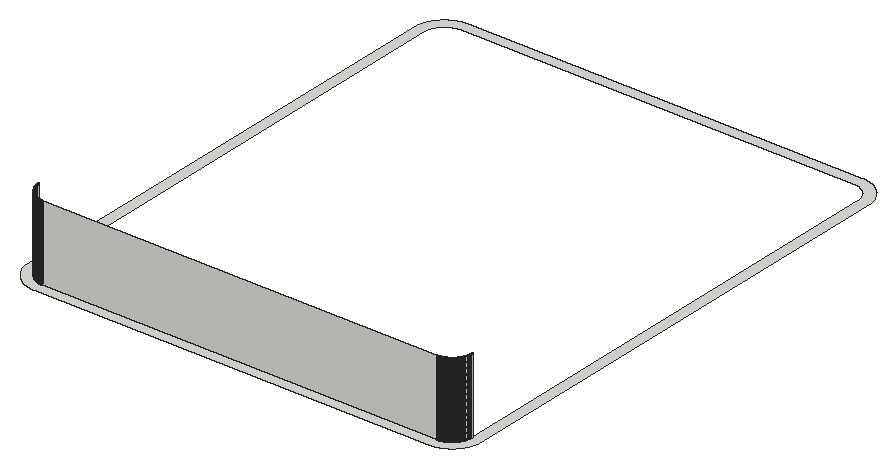
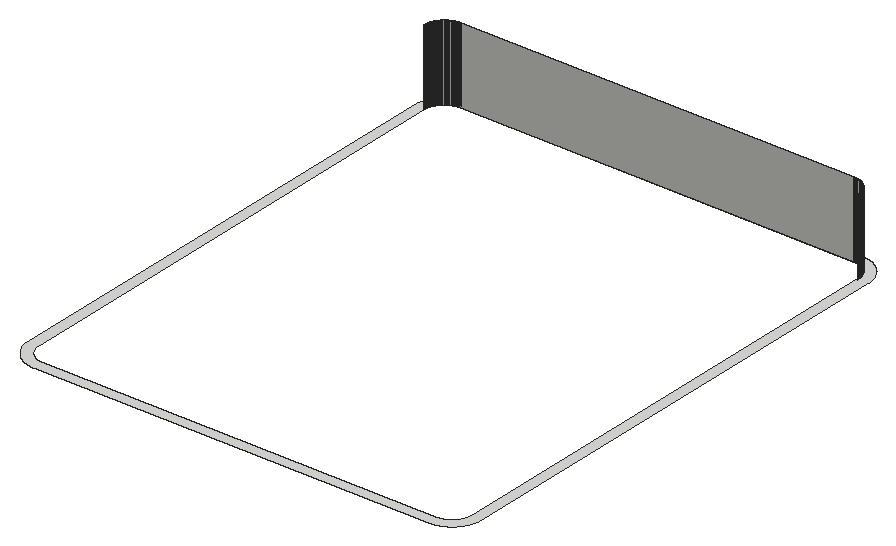
# SketchUp Ruby script. Lengths in inches.
U = 1.inch
M = Sketchup.active_model
def pt(a) = Geom::Point3d.new(a.map { |v| v * U })
def face(e, loops, mat)
  f = e.add_face(loops[0].map { |a| pt(a) })
  loops[1..].each { |l| e.add_face(l.map { |a| pt(a) }).erase! }
  f.material = f.back_material = mat if mat
  f
end
# faces: each face lists its corners as indices into pts; further lists are holes
def faces(e, pts, list, mat = nil) = list.each { |f| face(e, (f[0].is_a?(Array) ? f : [f]).map { |l| l.map { |i| pts[i] } }, mat) }
# xy, xz, yz: faces in a plane at the given z, y or x. An outline is a flat list of corners, or four numbers for a rectangle; further outlines are holes
def ring(l) = l.size == 4 ? [[l[0], l[1]], [l[2], l[1]], [l[2], l[3]], [l[0], l[3]]] : l.each_slice(2).to_a
def flat(e, list, mat, &to3) = list.each { |f| face(e, (f[0].is_a?(Array) ? f : [f]).map { |l| ring(l).map { |u, v| to3.(u, v) } }, mat) }
def xy(e, z, list, mat = nil) = flat(e, list, mat) { |x, y| [x, y, z] }
def xz(e, y, list, mat = nil) = flat(e, list, mat) { |x, z| [x, y, z] }
def yz(e, x, list, mat = nil) = flat(e, list, mat) { |y, z| [x, y, z] }
def lines(e, pts, list) = list.each { |a, b| e.add_line(pt(pts[a]), pt(pts[b])) }
# prism: a flat outline (further loops are holes) pulled along v
def prism(e, loops, v, mat = nil)
  f = face(e, loops, mat); d = Geom::Vector3d.new(v.map { |x| x * U })
  f.pushpull(f.normal.samedirection?(d) ? d.length : -d.length)
end
def box(e, o, s, mat = nil) = prism(e, [[o, [o[0] + s[0], o[1], o[2]], [o[0] + s[0], o[1] + s[1], o[2]], [o[0], o[1] + s[1], o[2]]]], [0, 0, s[2]], mat)
def at(x, y, z, deg = 0) = Geom::Transformation.translation(pt([x, y, z])) * Geom::Transformation.rotation(ORIGIN, Z_AXIS, deg.degrees)
def axes(o, x, y, z) = Geom::Transformation.new([*x, 0, *y, 0, *z, 0, *pt(o).to_a, 1])
def part(name) = M.definitions.add(name)
# library, detail: a bought-in or finely detailed component or shape, given as its bounding box
def library(name, o, s) = part(name).tap { |d| box(d.entities, o, s) }
def detail(e, o, s) = box(e.add_group.entities, o, s)
def put(e, d, t, mat = nil) = e.add_instance(d, t).tap { |i| i.material = mat if mat }
def group(e, t, mat = nil) = e.add_group.tap { |g| g.transformation = t; g.material = mat if mat }.entities
root = M.entities
M.materials.add("[Formica Graystone]").color = [224, 223, 219]
xy(root,392.82,[[[17.6875,229,174.3125,229,174.47,229.01,174.63,229.02,174.78,229.03,175.1,229.05,175.25,229.07,175.41,229.08,175.57,229.1,175.72,229.125,175.88,229.15,176.03,229.17,176.1875,229.2,176.34,229.23,176.49,229.26,176.65,229.3,176.8,229.33,176.95,229.37,177.11,229.41,177.41,229.49,177.86,229.64,178.01,229.6875,178.15,229.74,178.3,229.8,178.45,229.85,178.59,229.91,178.74,229.97,178.88,230.04,179.02,230.1,179.17,230.17,179.73,230.45,179.86,230.53,180,230.61,180.14,230.6875,180.27,230.77,180.4,230.85,180.54,230.9375,180.67,231.02,180.93,231.2,181.05,231.29,181.18,231.38,181.31,231.48,181.43,231.58,181.55,231.67,181.67,231.77,181.91,231.98,182.03,232.08,182.15,232.1875,182.26,232.3,182.375,232.4,182.49,232.51,182.6,232.625,182.7,232.74,182.8125,232.85,182.92,232.97,183.02,233.09,183.23,233.33,183.33,233.45,183.42,233.57,183.52,233.69,183.62,233.82,183.71,233.95,183.8,234.07,183.98,234.33,184.0625,234.46,184.15,234.6,184.23,234.73,184.3125,234.86,184.39,235,184.47,235.14,184.55,235.27,184.83,235.83,184.9,235.98,184.96,236.12,185.03,236.26,185.09,236.41,185.15,236.55,185.2,236.7,185.26,236.85,185.3125,236.99,185.36,237.14,185.51,237.59,185.59,237.89,185.63,238.05,185.67,238.2,185.7,238.35,185.74,238.51,185.77,238.66,185.8,238.8125,185.83,238.97,185.85,239.12,185.875,239.28,185.9,239.43,185.92,239.59,185.93,239.75,185.95,239.9,185.97,240.22,185.98,240.37,185.99,240.53,186,240.6875,186,432.3125,185.99,432.47,185.98,432.63,185.97,432.78,185.95,433.1,185.93,433.25,185.92,433.41,185.9,433.57,185.875,433.72,185.85,433.88,185.83,434.03,185.8,434.1875,185.77,434.34,185.74,434.49,185.7,434.65,185.67,434.8,185.63,434.95,185.59,435.11,185.51,435.41,185.36,435.86,185.3125,436.01,185.26,436.15,185.2,436.3,185.15,436.45,185.09,436.59,185.03,436.74,184.96,436.88,184.9,437.02,184.83,437.17,184.55,437.73,184.47,437.86,184.39,438,184.3125,438.14,184.23,438.27,184.15,438.4,184.0625,438.54,183.98,438.67,183.8,438.93,183.71,439.05,183.62,439.18,183.52,439.31,183.42,439.43,183.33,439.55,183.23,439.67,183.02,439.91,182.92,440.03,182.8125,440.15,182.7,440.26,182.6,440.375,182.49,440.49,182.375,440.6,182.26,440.7,182.15,440.8125,182.03,440.92,181.91,441.02,181.67,441.23,181.55,441.33,181.43,441.42,181.31,441.52,181.18,441.62,181.05,441.71,180.93,441.8,180.67,441.98,180.54,442.0625,180.4,442.15,180.27,442.23,180.14,442.3125,180,442.39,179.86,442.47,179.73,442.55,179.17,442.83,179.02,442.9,178.88,442.96,178.74,443.03,178.59,443.09,178.45,443.15,178.3,443.2,178.15,443.26,178.01,443.3125,177.86,443.36,177.41,443.51,177.11,443.59,176.95,443.63,176.8,443.67,176.65,443.7,176.49,443.74,176.34,443.77,176.1875,443.8,176.03,443.83,175.88,443.85,175.72,443.875,175.57,443.9,175.41,443.92,175.25,443.93,175.1,443.95,174.78,443.97,174.63,443.98,174.47,443.99,174.3125,444,17.6875,444,17.53,443.99,17.37,443.98,17.22,443.97,16.9,443.95,16.75,443.93,16.59,443.92,16.43,443.9,16.28,443.875,16.12,443.85,15.97,443.83,15.8125,443.8,15.66,443.77,15.51,443.74,15.35,443.7,15.2,443.67,15.05,443.63,14.89,443.59,14.59,443.51,14.14,443.36,13.99,443.3125,13.85,443.26,13.7,443.2,13.55,443.15,13.41,443.09,13.26,443.03,13.12,442.96,12.98,442.9,12.83,442.83,12.27,442.55,12.14,442.47,12,442.39,11.86,442.3125,11.73,442.23,11.6,442.15,11.46,442.0625,11.33,441.98,11.07,441.8,10.95,441.71,10.82,441.62,10.69,441.52,10.57,441.42,10.45,441.33,10.33,441.23,10.09,441.02,9.97,440.92,9.85,440.8125,9.74,440.7,9.625,440.6,9.51,440.49,9.4,440.375,9.3,440.26,9.1875,440.15,9.08,440.03,8.98,439.91,8.77,439.67,8.67,439.55,8.58,439.43,8.48,439.31,8.38,439.18,8.29,439.05,8.2,438.93,8.02,438.67,7.9375,438.54,7.85,438.4,7.77,438.27,7.6875,438.14,7.61,438,7.53,437.86,7.45,437.73,7.17,437.17,7.1,437.02,7.04,436.88,6.97,436.74,6.91,436.59,6.85,436.45,6.8,436.3,6.74,436.15,6.6875,436.01,6.64,435.86,6.49,435.41,6.41,435.11,6.37,434.95,6.33,434.8,6.3,434.65,6.26,434.49,6.23,434.34,6.2,434.1875,6.17,434.03,6.15,433.88,6.125,433.72,6.1,433.57,6.08,433.41,6.07,433.25,6.05,433.1,6.03,432.78,6.02,432.63,6.01,432.47,6,432.3125,6,240.6875,6.01,240.53,6.02,240.37,6.03,240.22,6.05,239.9,6.07,239.75,6.08,239.59,6.1,239.43,6.125,239.28,6.15,239.12,6.17,238.97,6.2,238.8125,6.23,238.66,6.26,238.51,6.3,238.35,6.33,238.2,6.37,238.05,6.41,237.89,6.49,237.59,6.64,237.14,6.6875,236.99,6.74,236.85,6.8,236.7,6.85,236.55,6.91,236.41,6.97,236.26,7.04,236.12,7.1,235.98,7.17,235.83,7.45,235.27,7.53,235.14,7.61,235,7.6875,234.86,7.77,234.73,7.85,234.6,7.9375,234.46,8.02,234.33,8.2,234.07,8.29,233.95,8.38,233.82,8.48,233.69,8.58,233.57,8.67,233.45,8.77,233.33,8.98,233.09,9.08,232.97,9.1875,232.85,9.3,232.74,9.4,232.625,9.51,232.51,9.625,232.4,9.74,232.3,9.85,232.1875,9.97,232.08,10.09,231.98,10.33,231.77,10.45,231.67,10.57,231.58,10.69,231.48,10.82,231.38,10.95,231.29,11.07,231.2,11.33,231.02,11.46,230.9375,11.6,230.85,11.73,230.77,11.86,230.6875,12,230.61,12.14,230.53,12.27,230.45,12.83,230.17,12.98,230.1,13.12,230.04,13.26,229.97,13.41,229.91,13.55,229.85,13.7,229.8,13.85,229.74,13.99,229.6875,14.14,229.64,14.59,229.49,14.89,229.41,15.05,229.37,15.2,229.33,15.35,229.3,15.51,229.26,15.66,229.23,15.8125,229.2,15.97,229.17,16.12,229.15,16.28,229.125,16.43,229.1,16.59,229.08,16.75,229.07,16.9,229.05,17.22,229.03,17.37,229.02,17.53,229.01],[17.79,233,17.6875,233.01,17.58,233.01,17.48,233.02,17.37,233.02,17.27,233.03,17.16,233.04,17.06,233.06,16.96,233.07,16.85,233.08,16.65,233.12,16.54,233.13,16.4375,233.15,16.34,233.17,16.23,233.2,16.13,233.22,16.03,233.25,15.93,233.27,15.43,233.42,15.33,233.46,15.23,233.49,15.13,233.53,15.04,233.57,14.9375,233.61,14.84,233.65,14.75,233.69,14.65,233.73,14.56,233.78,14.46,233.83,14.37,233.87,14.28,233.92,14.18,233.97,14,234.07,13.82,234.18,13.73,234.23,13.64,234.29,13.56,234.35,13.38,234.47,13.3,234.53,13.21,234.59,13.13,234.65,13.05,234.72,12.97,234.78,12.88,234.85,12.8,234.92,12.73,234.99,12.65,235.05,12.49,235.2,12.42,235.27,12.34,235.34,12.27,235.42,12.2,235.49,12.05,235.65,11.99,235.73,11.92,235.8,11.85,235.88,11.78,235.97,11.72,236.05,11.65,236.13,11.59,236.21,11.53,236.3,11.47,236.38,11.35,236.56,11.29,236.64,11.23,236.73,11.18,236.82,11.07,237,10.97,237.18,10.92,237.28,10.87,237.37,10.83,237.46,10.78,237.56,10.73,237.65,10.69,237.75,10.65,237.84,10.61,237.9375,10.57,238.04,10.53,238.13,10.49,238.23,10.46,238.33,10.42,238.43,10.27,238.93,10.25,239.03,10.22,239.13,10.2,239.23,10.17,239.34,10.15,239.4375,10.13,239.54,10.12,239.65,10.08,239.85,10.07,239.96,10.06,240.06,10.04,240.16,10.03,240.27,10.02,240.37,10.02,240.48,10.01,240.58,10.01,240.6875,10,240.79,10,432.21,10.01,432.3125,10.01,432.42,10.02,432.52,10.02,432.63,10.03,432.73,10.04,432.84,10.06,432.94,10.07,433.04,10.08,433.15,10.12,433.35,10.13,433.46,10.15,433.5625,10.17,433.66,10.2,433.77,10.22,433.87,10.25,433.97,10.27,434.07,10.42,434.57,10.46,434.67,10.49,434.77,10.53,434.87,10.57,434.96,10.61,435.0625,10.65,435.16,10.69,435.25,10.73,435.35,10.78,435.44,10.83,435.54,10.87,435.63,10.92,435.72,10.97,435.82,11.07,436,11.18,436.18,11.23,436.27,11.29,436.36,11.35,436.44,11.47,436.62,11.53,436.7,11.59,436.79,11.65,436.87,11.72,436.95,11.78,437.03,11.85,437.12,11.92,437.2,11.99,437.27,12.05,437.35,12.2,437.51,12.27,437.58,12.34,437.66,12.42,437.73,12.49,437.8,12.65,437.95,12.73,438.01,12.8,438.08,12.88,438.15,12.97,438.22,13.05,438.28,13.13,438.35,13.21,438.41,13.3,438.47,13.38,438.53,13.56,438.65,13.64,438.71,13.73,438.77,13.82,438.82,14,438.93,14.18,439.03,14.28,439.08,14.37,439.13,14.46,439.17,14.56,439.22,14.65,439.27,14.75,439.31,14.84,439.35,14.9375,439.39,15.04,439.43,15.13,439.47,15.23,439.51,15.33,439.54,15.43,439.58,15.93,439.73,16.03,439.75,16.13,439.78,16.23,439.8,16.34,439.83,16.4375,439.85,16.54,439.87,16.65,439.88,16.85,439.92,16.96,439.93,17.06,439.94,17.16,439.96,17.27,439.97,17.37,439.98,17.48,439.98,17.58,439.99,17.6875,439.99,17.79,440,174.21,440,174.3125,439.99,174.42,439.99,174.52,439.98,174.63,439.98,174.73,439.97,174.84,439.96,174.94,439.94,175.04,439.93,175.15,439.92,175.35,439.88,175.46,439.87,175.5625,439.85,175.66,439.83,175.77,439.8,175.87,439.78,175.97,439.75,176.07,439.73,176.57,439.58,176.67,439.54,176.77,439.51,176.87,439.47,176.96,439.43,177.0625,439.39,177.16,439.35,177.25,439.31,177.35,439.27,177.44,439.22,177.54,439.17,177.63,439.13,177.72,439.08,177.82,439.03,178,438.93,178.18,438.82,178.27,438.77,178.36,438.71,178.44,438.65,178.62,438.53,178.7,438.47,178.79,438.41,178.87,438.35,178.95,438.28,179.03,438.22,179.12,438.15,179.2,438.08,179.27,438.01,179.35,437.95,179.51,437.8,179.58,437.73,179.66,437.66,179.73,437.58,179.8,437.51,179.95,437.35,180.01,437.27,180.08,437.2,180.15,437.12,180.22,437.03,180.28,436.95,180.35,436.87,180.41,436.79,180.47,436.7,180.53,436.62,180.65,436.44,180.71,436.36,180.77,436.27,180.82,436.18,180.93,436,181.03,435.82,181.08,435.72,181.13,435.63,181.17,435.54,181.22,435.44,181.27,435.35,181.31,435.25,181.35,435.16,181.39,435.0625,181.43,434.96,181.47,434.87,181.51,434.77,181.54,434.67,181.58,434.57,181.73,434.07,181.75,433.97,181.78,433.87,181.8,433.77,181.83,433.66,181.85,433.5625,181.87,433.46,181.88,433.35,181.92,433.15,181.93,433.04,181.94,432.94,181.96,432.84,181.97,432.73,181.98,432.63,181.98,432.52,181.99,432.42,181.99,432.3125,182,432.21,182,240.79,181.99,240.6875,181.99,240.58,181.98,240.48,181.98,240.37,181.97,240.27,181.96,240.16,181.94,240.06,181.93,239.96,181.92,239.85,181.88,239.65,181.87,239.54,181.85,239.4375,181.83,239.34,181.8,239.23,181.78,239.13,181.75,239.03,181.73,238.93,181.58,238.43,181.54,238.33,181.51,238.23,181.47,238.13,181.43,238.04,181.39,237.9375,181.35,237.84,181.31,237.75,181.27,237.65,181.22,237.56,181.17,237.46,181.13,237.37,181.08,237.28,181.03,237.18,180.93,237,180.82,236.82,180.77,236.73,180.71,236.64,180.65,236.56,180.53,236.38,180.47,236.3,180.41,236.21,180.35,236.13,180.28,236.05,180.22,235.97,180.15,235.88,180.08,235.8,180.01,235.73,179.95,235.65,179.8,235.49,179.73,235.42,179.66,235.34,179.58,235.27,179.51,235.2,179.35,235.05,179.27,234.99,179.2,234.92,179.12,234.85,179.03,234.78,178.95,234.72,178.87,234.65,178.79,234.59,178.7,234.53,178.62,234.47,178.44,234.35,178.36,234.29,178.27,234.23,178.18,234.18,178,234.07,177.82,233.97,177.72,233.92,177.63,233.87,177.54,233.83,177.44,233.78,177.35,233.73,177.25,233.69,177.16,233.65,177.0625,233.61,176.96,233.57,176.87,233.53,176.77,233.49,176.67,233.46,176.57,233.42,176.07,233.27,175.97,233.25,175.87,233.22,175.77,233.2,175.66,233.17,175.5625,233.15,175.46,233.13,175.35,233.12,175.15,233.08,175.04,233.07,174.94,233.06,174.84,233.04,174.73,233.03,174.63,233.02,174.52,233.02,174.42,233.01,174.3125,233.01,174.21,233]]],"[Formica Graystone]")
xz(root,233,[[17.79,392.82,17.9,422.82],[17.9,392.82,18,422.82],[18,392.82,174,422.82],[174,392.82,174.1,422.82],[174.1,392.82,174.21,422.82]],"[Formica Graystone]")
xz(root,233.01,[[17.58,392.82,17.6875,422.82],[174.3125,392.82,174.42,422.82]],"[Formica Graystone]")
xz(root,233.02,[[17.37,392.82,17.48,422.82],[174.52,392.82,174.63,422.82]],"[Formica Graystone]")
yz(root,10,[[240.79,392.82,240.9,422.82],[240.9,392.82,241,422.82]],"[Formica Graystone]")
yz(root,10.01,[[240.58,392.82,240.6875,422.82]],"[Formica Graystone]")
yz(root,10.02,[[240.37,392.82,240.48,422.82]],"[Formica Graystone]")
yz(root,181.98,[[240.37,392.82,240.48,422.82]],"[Formica Graystone]")
yz(root,181.99,[[240.58,392.82,240.6875,422.82]],"[Formica Graystone]")
yz(root,182,[[240.79,392.82,240.9,422.82],[240.9,392.82,241,422.82]],"[Formica Graystone]")
p = [[17.06,233.06,392.82],[17.16,233.04,392.82],[17.16,233.04,422.82],[17.06,233.06,422.82],[17.27,233.03,392.82],[17.27,233.03,422.82],
  [17.37,233.02,392.82],[17.37,233.02,422.82],[17.48,233.02,392.82],[17.58,233.01,392.82],[17.58,233.01,422.82],[17.48,233.02,422.82],
  [17.6875,233.01,392.82],[17.79,233,392.82],[17.79,233,422.82],[17.6875,233.01,422.82],[174.21,233,392.82],[174.3125,233.01,392.82],
  [174.3125,233.01,422.82],[174.21,233,422.82],[174.42,233.01,392.82],[174.52,233.02,392.82],[174.52,233.02,422.82],[174.42,233.01,422.82],
  [174.63,233.02,392.82],[174.73,233.03,392.82],[174.73,233.03,422.82],[174.63,233.02,422.82],[174.84,233.04,392.82],[174.84,233.04,422.82],
  [174.94,233.06,392.82],[174.94,233.06,422.82],[16.4375,233.15,392.82],[16.54,233.13,392.82],[16.54,233.13,422.82],[16.4375,233.15,422.82],
  [16.65,233.12,392.82],[16.65,233.12,422.82],[16.75,233.1,392.82],[16.75,233.1,422.82],[16.85,233.08,392.82],[16.85,233.08,422.82],
  [16.96,233.07,392.82],[16.96,233.07,422.82],[175.04,233.07,392.82],[175.04,233.07,422.82],[175.15,233.08,392.82],[175.15,233.08,422.82],
  [175.25,233.1,392.82],[175.25,233.1,422.82],[175.35,233.12,392.82],[175.35,233.12,422.82],[175.46,233.13,392.82],[175.46,233.13,422.82],
  [175.5625,233.15,392.82],[175.5625,233.15,422.82],[15.93,233.27,392.82],[16.03,233.25,392.82],[16.03,233.25,422.82],[15.93,233.27,422.82],
  [16.13,233.22,392.82],[16.13,233.22,422.82],[16.23,233.2,392.82],[16.23,233.2,422.82],[16.34,233.17,392.82],[16.34,233.17,422.82],
  [175.66,233.17,392.82],[175.66,233.17,422.82],[175.77,233.2,392.82],[175.77,233.2,422.82],[175.87,233.22,392.82],[175.87,233.22,422.82],
  [175.97,233.25,392.82],[175.97,233.25,422.82],[176.07,233.27,392.82],[176.07,233.27,422.82],[15.63,233.36,392.82],[15.73,233.33,392.82],
  [15.73,233.33,422.82],[15.63,233.36,422.82],[15.83,233.3,392.82],[15.83,233.3,422.82],[176.17,233.3,392.82],[176.17,233.3,422.82],
  [176.27,233.33,392.82],[176.27,233.33,422.82],[176.37,233.36,392.82],[176.37,233.36,422.82],[15.33,233.46,392.82],[15.43,233.42,392.82],
  [15.43,233.42,422.82],[15.33,233.46,422.82],[15.53,233.39,392.82],[15.53,233.39,422.82],[176.47,233.39,392.82],[176.47,233.39,422.82],
  [176.57,233.42,392.82],[176.57,233.42,422.82],[176.67,233.46,392.82],[176.67,233.46,422.82],[15.04,233.57,392.82],[15.13,233.53,392.82],
  [15.13,233.53,422.82],[15.04,233.57,422.82],[15.23,233.49,392.82],[15.23,233.49,422.82],[176.77,233.49,392.82],[176.77,233.49,422.82],
  [176.87,233.53,392.82],[176.87,233.53,422.82],[176.96,233.57,392.82],[176.96,233.57,422.82],[14.75,233.69,392.82],[14.84,233.65,392.82],
  [14.84,233.65,422.82],[14.75,233.69,422.82],[14.9375,233.61,392.82],[14.9375,233.61,422.82],[177.0625,233.61,392.82],[177.0625,233.61,422.82],
  [177.16,233.65,392.82],[177.16,233.65,422.82],[177.25,233.69,392.82],[177.25,233.69,422.82],[14.56,233.78,392.82],[14.65,233.73,392.82],
  [14.65,233.73,422.82],[14.56,233.78,422.82],[177.35,233.73,392.82],[177.35,233.73,422.82],[177.44,233.78,392.82],[177.44,233.78,422.82],
  [14.37,233.87,392.82],[14.46,233.83,392.82],[14.46,233.83,422.82],[14.37,233.87,422.82],[177.54,233.83,392.82],[177.54,233.83,422.82],
  [177.63,233.87,392.82],[177.63,233.87,422.82],[14.18,233.97,392.82],[14.28,233.92,392.82],[14.28,233.92,422.82],[14.18,233.97,422.82],
  [177.72,233.92,392.82],[177.72,233.92,422.82],[177.82,233.97,392.82],[177.82,233.97,422.82],[14,234.07,392.82],[14.09,234.02,392.82],
  [14.09,234.02,422.82],[14,234.07,422.82],[177.91,234.02,392.82],[177.91,234.02,422.82],[178,234.07,392.82],[178,234.07,422.82],
  [13.82,234.18,392.82],[13.91,234.125,392.82],[13.91,234.125,422.82],[13.82,234.18,422.82],[178.09,234.125,392.82],[178.09,234.125,422.82],
  [178.18,234.18,392.82],[178.18,234.18,422.82],[13.64,234.29,392.82],[13.73,234.23,392.82],[13.73,234.23,422.82],[13.64,234.29,422.82],
  [178.27,234.23,392.82],[178.27,234.23,422.82],[178.36,234.29,392.82],[178.36,234.29,422.82],[13.47,234.41,392.82],[13.56,234.35,392.82],
  [13.56,234.35,422.82],[13.47,234.41,422.82],[178.44,234.35,392.82],[178.44,234.35,422.82],[178.53,234.41,392.82],[178.53,234.41,422.82],
  [13.38,234.47,392.82],[13.38,234.47,422.82],[178.62,234.47,392.82],[178.62,234.47,422.82],[13.21,234.59,392.82],[13.3,234.53,392.82],
  [13.3,234.53,422.82],[13.21,234.59,422.82],[178.7,234.53,392.82],[178.7,234.53,422.82],[178.79,234.59,392.82],[178.79,234.59,422.82],
  [13.13,234.65,392.82],[13.13,234.65,422.82],[178.87,234.65,392.82],[178.87,234.65,422.82],[13.05,234.72,392.82],[13.05,234.72,422.82],
  [12.97,234.78,392.82],[12.97,234.78,422.82],[178.95,234.72,392.82],[178.95,234.72,422.82],[179.03,234.78,392.82],[179.03,234.78,422.82],
  [12.8,234.92,392.82],[12.88,234.85,392.82],[12.88,234.85,422.82],[12.8,234.92,422.82],[179.12,234.85,392.82],[179.12,234.85,422.82],
  [179.2,234.92,392.82],[179.2,234.92,422.82],[12.73,234.99,392.82],[12.73,234.99,422.82],[179.27,234.99,392.82],[179.27,234.99,422.82],
  [12.65,235.05,392.82],[12.65,235.05,422.82],[179.35,235.05,392.82],[179.35,235.05,422.82],[12.49,235.2,392.82],[12.57,235.125,392.82],
  [12.57,235.125,422.82],[12.49,235.2,422.82],[179.43,235.125,392.82],[179.43,235.125,422.82],[179.51,235.2,392.82],[179.51,235.2,422.82],
  [12.42,235.27,392.82],[12.42,235.27,422.82],[179.58,235.27,392.82],[179.58,235.27,422.82],[12.34,235.34,392.82],[12.34,235.34,422.82],
  [12.27,235.42,392.82],[12.27,235.42,422.82],[179.66,235.34,392.82],[179.66,235.34,422.82],[179.73,235.42,392.82],[179.73,235.42,422.82],
  [12.2,235.49,392.82],[12.2,235.49,422.82],[179.8,235.49,392.82],[179.8,235.49,422.82],[12.125,235.57,392.82],[12.125,235.57,422.82],
  [179.875,235.57,392.82],[179.875,235.57,422.82],[11.99,235.73,392.82],[12.05,235.65,392.82],[12.05,235.65,422.82],[11.99,235.73,422.82],
  [179.95,235.65,392.82],[179.95,235.65,422.82],[180.01,235.73,392.82],[180.01,235.73,422.82],[11.92,235.8,392.82],[11.92,235.8,422.82],
  [180.08,235.8,392.82],[180.08,235.8,422.82],[11.85,235.88,392.82],[11.85,235.88,422.82],[180.15,235.88,392.82],[180.15,235.88,422.82],
  [11.78,235.97,392.82],[11.78,235.97,422.82],[180.22,235.97,392.82],[180.22,235.97,422.82],[11.72,236.05,392.82],[11.72,236.05,422.82],
  [11.65,236.13,392.82],[11.65,236.13,422.82],[180.28,236.05,392.82],[180.28,236.05,422.82],[180.35,236.13,392.82],[180.35,236.13,422.82],
  [11.59,236.21,392.82],[11.59,236.21,422.82],[180.41,236.21,392.82],[180.41,236.21,422.82],[11.53,236.3,392.82],[11.53,236.3,422.82],
  [180.47,236.3,392.82],[180.47,236.3,422.82],[11.47,236.38,392.82],[11.47,236.38,422.82],[180.53,236.38,392.82],[180.53,236.38,422.82],
  [11.41,236.47,392.82],[11.41,236.47,422.82],[180.59,236.47,392.82],[180.59,236.47,422.82],[11.35,236.56,392.82],[11.35,236.56,422.82],
  [180.65,236.56,392.82],[180.65,236.56,422.82],[11.23,236.73,392.82],[11.29,236.64,392.82],[11.29,236.64,422.82],[11.23,236.73,422.82],
  [180.71,236.64,392.82],[180.71,236.64,422.82],[180.77,236.73,392.82],[180.77,236.73,422.82],[11.18,236.82,392.82],[11.18,236.82,422.82],
  [180.82,236.82,392.82],[180.82,236.82,422.82],[11.125,236.91,392.82],[11.125,236.91,422.82],[180.875,236.91,392.82],[180.875,236.91,422.82],
  [11.07,237,392.82],[11.07,237,422.82],[180.93,237,392.82],[180.93,237,422.82],[11.02,237.09,392.82],[11.02,237.09,422.82],
  [180.98,237.09,392.82],[180.98,237.09,422.82],[10.97,237.18,392.82],[10.97,237.18,422.82],[181.03,237.18,392.82],[181.03,237.18,422.82],
  [10.92,237.28,392.82],[10.92,237.28,422.82],[181.08,237.28,392.82],[181.08,237.28,422.82],[10.87,237.37,392.82],[10.87,237.37,422.82],
  [181.13,237.37,392.82],[181.13,237.37,422.82],[10.83,237.46,392.82],[10.83,237.46,422.82],[181.17,237.46,392.82],[181.17,237.46,422.82],
  [10.78,237.56,392.82],[10.78,237.56,422.82],[181.22,237.56,392.82],[181.22,237.56,422.82],[10.73,237.65,392.82],[10.73,237.65,422.82],
  [181.27,237.65,392.82],[181.27,237.65,422.82],[10.65,237.84,392.82],[10.69,237.75,392.82],[10.69,237.75,422.82],[10.65,237.84,422.82],
  [181.31,237.75,392.82],[181.31,237.75,422.82],[181.35,237.84,392.82],[181.35,237.84,422.82],[10.61,237.9375,392.82],[10.61,237.9375,422.82],
  [181.39,237.9375,392.82],[181.39,237.9375,422.82],[10.57,238.04,392.82],[10.57,238.04,422.82],[181.43,238.04,392.82],[181.43,238.04,422.82],
  [10.53,238.13,392.82],[10.53,238.13,422.82],[181.47,238.13,392.82],[181.47,238.13,422.82],[10.49,238.23,392.82],[10.49,238.23,422.82],
  [181.51,238.23,392.82],[181.51,238.23,422.82],[10.46,238.33,392.82],[10.46,238.33,422.82],[181.54,238.33,392.82],[181.54,238.33,422.82],
  [10.42,238.43,392.82],[10.42,238.43,422.82],[181.58,238.43,392.82],[181.58,238.43,422.82],[10.39,238.53,392.82],[10.39,238.53,422.82],
  [181.61,238.53,392.82],[181.61,238.53,422.82],[10.36,238.63,392.82],[10.36,238.63,422.82],[181.64,238.63,392.82],[181.64,238.63,422.82],
  [10.33,238.73,392.82],[10.33,238.73,422.82],[181.67,238.73,392.82],[181.67,238.73,422.82],[10.3,238.83,392.82],[10.3,238.83,422.82],
  [181.7,238.83,392.82],[181.7,238.83,422.82],[10.27,238.93,392.82],[10.27,238.93,422.82],[181.73,238.93,392.82],[181.73,238.93,422.82],
  [10.25,239.03,392.82],[10.25,239.03,422.82],[181.75,239.03,392.82],[181.75,239.03,422.82],[10.22,239.13,392.82],[10.22,239.13,422.82],
  [181.78,239.13,392.82],[181.78,239.13,422.82],[10.2,239.23,392.82],[10.2,239.23,422.82],[181.8,239.23,392.82],[181.8,239.23,422.82],
  [10.17,239.34,392.82],[10.17,239.34,422.82],[181.83,239.34,392.82],[181.83,239.34,422.82],[10.15,239.4375,392.82],[10.15,239.4375,422.82],
  [181.85,239.4375,392.82],[181.85,239.4375,422.82],[10.13,239.54,392.82],[10.13,239.54,422.82],[181.87,239.54,392.82],[181.87,239.54,422.82],
  [10.12,239.65,392.82],[10.12,239.65,422.82],[181.88,239.65,392.82],[181.88,239.65,422.82],[10.1,239.75,392.82],[10.1,239.75,422.82],
  [181.9,239.75,392.82],[181.9,239.75,422.82],[10.08,239.85,392.82],[10.08,239.85,422.82],[181.92,239.85,392.82],[181.92,239.85,422.82],
  [10.07,239.96,392.82],[10.07,239.96,422.82],[181.93,239.96,392.82],[181.93,239.96,422.82],[10.06,240.06,392.82],[10.06,240.06,422.82],
  [181.94,240.06,392.82],[181.94,240.06,422.82],[10.04,240.16,392.82],[10.04,240.16,422.82],[181.96,240.16,392.82],[181.96,240.16,422.82],
  [10.03,240.27,392.82],[10.03,240.27,422.82],[181.97,240.27,392.82],[181.97,240.27,422.82],[10.02,240.37,392.82],[10.02,240.37,422.82],
  [181.98,240.37,392.82],[181.98,240.37,422.82],[10.01,240.58,392.82],[10.02,240.48,392.82],[10.02,240.48,422.82],[10.01,240.58,422.82],
  [181.98,240.48,392.82],[181.99,240.58,392.82],[181.99,240.58,422.82],[181.98,240.48,422.82],[10,240.79,392.82],[10.01,240.6875,392.82],
  [10.01,240.6875,422.82],[10,240.79,422.82],[181.99,240.6875,392.82],[182,240.79,392.82],[182,240.79,422.82],[181.99,240.6875,422.82]]
faces(root,p,[[0,1,2,3],[1,4,5,2],[4,6,7,5],[8,9,10,11],[12,13,14,15],[16,17,18,19],[20,21,22,23],[24,25,26,27],
  [25,28,29,26],[28,30,31,29],[32,33,34,35],[33,36,37,34],[36,38,39,37],[38,40,41,39],[40,42,43,41],[42,0,3,43],
  [30,44,45,31],[44,46,47,45],[46,48,49,47],[48,50,51,49],[50,52,53,51],[52,54,55,53],[56,57,58,59],[57,60,61,58],
  [60,62,63,61],[62,64,65,63],[64,32,35,65],[54,66,67,55],[66,68,69,67],[68,70,71,69],[70,72,73,71],[72,74,75,73],
  [76,77,78,79],[77,80,81,78],[80,56,59,81],[74,82,83,75],[82,84,85,83],[84,86,87,85],[88,89,90,91],[89,92,93,90],
  [92,76,79,93],[86,94,95,87],[94,96,97,95],[96,98,99,97],[100,101,102,103],[101,104,105,102],[104,88,91,105],[98,106,107,99],
  [106,108,109,107],[108,110,111,109],[112,113,114,115],[113,116,117,114],[116,100,103,117],[110,118,119,111],[118,120,121,119],[120,122,123,121],
  [124,125,126,127],[125,112,115,126],[122,128,129,123],[128,130,131,129],[132,133,134,135],[133,124,127,134],[130,136,137,131],[136,138,139,137],
  [140,141,142,143],[141,132,135,142],[138,144,145,139],[144,146,147,145],[148,149,150,151],[149,140,143,150],[146,152,153,147],[152,154,155,153],
  [156,157,158,159],[157,148,151,158],[154,160,161,155],[160,162,163,161],[164,165,166,167],[165,156,159,166],[162,168,169,163],[168,170,171,169],
  [172,173,174,175],[173,164,167,174],[170,176,177,171],[176,178,179,177],[180,172,175,181],[178,182,183,179],[184,185,186,187],[185,180,181,186],
  [182,188,189,183],[188,190,191,189],[192,184,187,193],[190,194,195,191],[196,192,193,197],[198,196,197,199],[194,200,201,195],[200,202,203,201],
  [204,205,206,207],[205,198,199,206],[202,208,209,203],[208,210,211,209],[212,204,207,213],[210,214,215,211],[216,212,213,217],[214,218,219,215],
  [220,221,222,223],[221,216,217,222],[218,224,225,219],[224,226,227,225],[228,220,223,229],[226,230,231,227],[232,228,229,233],[234,232,233,235],
  [230,236,237,231],[236,238,239,237],[240,234,235,241],[238,242,243,239],[244,240,241,245],[242,246,247,243],[248,249,250,251],[249,244,245,250],
  [246,252,253,247],[252,254,255,253],[256,248,251,257],[254,258,259,255],[260,256,257,261],[258,262,263,259],[264,260,261,265],[262,266,267,263],
  [268,264,265,269],[270,268,269,271],[266,272,273,267],[272,274,275,273],[276,270,271,277],[274,278,279,275],[280,276,277,281],[278,282,283,279],
  [284,280,281,285],[282,286,287,283],[288,284,285,289],[286,290,291,287],[292,288,289,293],[290,294,295,291],[296,297,298,299],[297,292,293,298],
  [294,300,301,295],[300,302,303,301],[304,296,299,305],[302,306,307,303],[308,304,305,309],[306,310,311,307],[312,308,309,313],[310,314,315,311],
  [316,312,313,317],[314,318,319,315],[320,316,317,321],[318,322,323,319],[324,320,321,325],[322,326,327,323],[328,324,325,329],[326,330,331,327],
  [332,328,329,333],[330,334,335,331],[336,332,333,337],[334,338,339,335],[340,336,337,341],[338,342,343,339],[344,345,346,347],[345,340,341,346],
  [342,348,349,343],[348,350,351,349],[352,344,347,353],[350,354,355,351],[356,352,353,357],[354,358,359,355],[360,356,357,361],[358,362,363,359],
  [364,360,361,365],[362,366,367,363],[368,364,365,369],[366,370,371,367],[372,368,369,373],[370,374,375,371],[376,372,373,377],[374,378,379,375],
  [380,376,377,381],[378,382,383,379],[384,380,381,385],[382,386,387,383],[388,384,385,389],[386,390,391,387],[392,388,389,393],[390,394,395,391],
  [396,392,393,397],[394,398,399,395],[400,396,397,401],[398,402,403,399],[404,400,401,405],[402,406,407,403],[408,404,405,409],[406,410,411,407],
  [412,408,409,413],[410,414,415,411],[416,412,413,417],[414,418,419,415],[420,416,417,421],[418,422,423,419],[424,420,421,425],[422,426,427,423],
  [428,424,425,429],[426,430,431,427],[432,428,429,433],[430,434,435,431],[436,432,433,437],[434,438,439,435],[440,436,437,441],[438,442,443,439],
  [444,440,441,445],[442,446,447,443],[448,444,445,449],[446,450,451,447],[452,453,454,455],[456,457,458,459],[460,461,462,463],[464,465,466,467]],"[Formica Graystone]")
